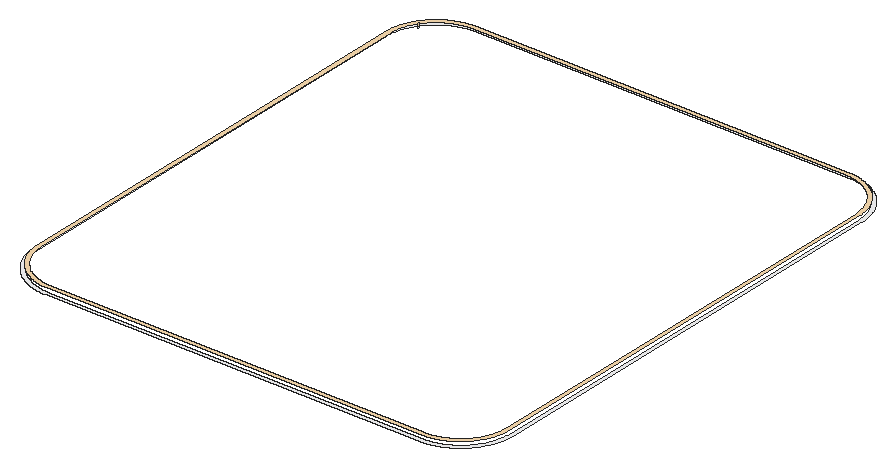
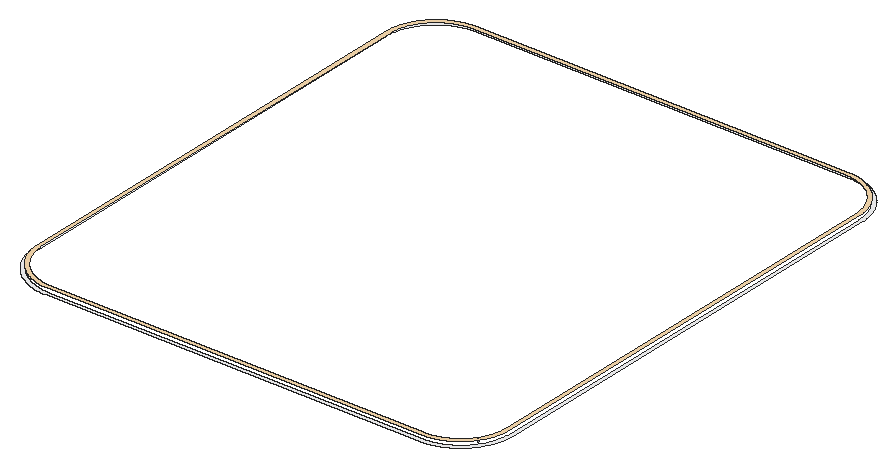
# SketchUp Ruby script. Lengths in inches.
U = 1.inch
M = Sketchup.active_model
def pt(a) = Geom::Point3d.new(a.map { |v| v * U })
def face(e, loops, mat)
  f = e.add_face(loops[0].map { |a| pt(a) })
  loops[1..].each { |l| e.add_face(l.map { |a| pt(a) }).erase! }
  f.material = f.back_material = mat if mat
  f
end
# faces: each face lists its corners as indices into pts; further lists are holes
def faces(e, pts, list, mat = nil) = list.each { |f| face(e, (f[0].is_a?(Array) ? f : [f]).map { |l| l.map { |i| pts[i] } }, mat) }
# xy, xz, yz: faces in a plane at the given z, y or x. An outline is a flat list of corners, or four numbers for a rectangle; further outlines are holes
def ring(l) = l.size == 4 ? [[l[0], l[1]], [l[2], l[1]], [l[2], l[3]], [l[0], l[3]]] : l.each_slice(2).to_a
def flat(e, list, mat, &to3) = list.each { |f| face(e, (f[0].is_a?(Array) ? f : [f]).map { |l| ring(l).map { |u, v| to3.(u, v) } }, mat) }
def xy(e, z, list, mat = nil) = flat(e, list, mat) { |x, y| [x, y, z] }
def xz(e, y, list, mat = nil) = flat(e, list, mat) { |x, z| [x, y, z] }
def yz(e, x, list, mat = nil) = flat(e, list, mat) { |y, z| [x, y, z] }
def lines(e, pts, list) = list.each { |a, b| e.add_line(pt(pts[a]), pt(pts[b])) }
# prism: a flat outline (further loops are holes) pulled along v
def prism(e, loops, v, mat = nil)
  f = face(e, loops, mat); d = Geom::Vector3d.new(v.map { |x| x * U })
  f.pushpull(f.normal.samedirection?(d) ? d.length : -d.length)
end
def box(e, o, s, mat = nil) = prism(e, [[o, [o[0] + s[0], o[1], o[2]], [o[0] + s[0], o[1] + s[1], o[2]], [o[0], o[1] + s[1], o[2]]]], [0, 0, s[2]], mat)
def at(x, y, z, deg = 0) = Geom::Transformation.translation(pt([x, y, z])) * Geom::Transformation.rotation(ORIGIN, Z_AXIS, deg.degrees)
def axes(o, x, y, z) = Geom::Transformation.new([*x, 0, *y, 0, *z, 0, *pt(o).to_a, 1])
def part(name) = M.definitions.add(name)
# library, detail: a bought-in or finely detailed component or shape, given as its bounding box
def library(name, o, s) = part(name).tap { |d| box(d.entities, o, s) }
def detail(e, o, s) = box(e.add_group.entities, o, s)
def put(e, d, t, mat = nil) = e.add_instance(d, t).tap { |i| i.material = mat if mat }
def group(e, t, mat = nil) = e.add_group.tap { |g| g.transformation = t; g.material = mat if mat }.entities
root = M.entities
M.materials.add("False Ceiling Light").color = [254, 223, 179]
M.materials.add("[Quartz Light Grey]").color = [251, 251, 252]
xy(root,115.32,[[[56.8,62.5,165.2,62.5,165.41,62.51,165.61,62.51,165.8125,62.52,166.01,62.53,166.22,62.55,166.42,62.56,166.62,62.58,166.82,62.61,167.02,62.63,167.42,62.69,167.625,62.72,167.82,62.76,168.42,62.88,168.82,62.98,169.01,63.03,169.21,63.08,169.4,63.14,169.6,63.2,169.98,63.32,170.74,63.6,171.12,63.76,171.3,63.84,171.49,63.92,171.67,64.01,171.86,64.1,172.04,64.1875,172.22,64.28,172.4,64.38,172.57,64.48,172.93,64.68,173.1,64.78,173.61,65.11,173.78,65.23,173.95,65.34,174.27,65.58,174.4375,65.7,174.75,65.95,175.07,66.21,175.22,66.35,175.37,66.48,175.82,66.9,176.1,67.18,176.52,67.63,176.65,67.78,176.79,67.93,177.05,68.25,177.3,68.5625,177.42,68.73,177.66,69.05,177.77,69.22,177.89,69.39,178.22,69.9,178.32,70.07,178.52,70.43,178.62,70.6,178.72,70.78,178.8125,70.96,178.9,71.14,178.99,71.33,179.08,71.51,179.16,71.7,179.24,71.88,179.4,72.26,179.68,73.02,179.8,73.4,179.86,73.6,179.92,73.79,179.97,73.99,180.02,74.18,180.12,74.58,180.24,75.18,180.28,75.375,180.31,75.58,180.37,75.98,180.39,76.18,180.42,76.38,180.44,76.58,180.45,76.78,180.47,76.99,180.48,77.1875,180.49,77.39,180.49,77.59,180.5,77.8,180.5,204.2,180.49,204.41,180.49,204.61,180.48,204.8125,180.47,205.01,180.45,205.22,180.44,205.42,180.42,205.62,180.39,205.82,180.37,206.02,180.31,206.42,180.28,206.625,180.24,206.82,180.12,207.42,180.02,207.82,179.97,208.01,179.92,208.21,179.86,208.4,179.8,208.6,179.68,208.98,179.4,209.74,179.24,210.12,179.16,210.3,179.08,210.49,178.99,210.67,178.9,210.86,178.8125,211.04,178.72,211.22,178.62,211.4,178.52,211.57,178.32,211.93,178.22,212.1,177.89,212.61,177.77,212.78,177.66,212.95,177.42,213.27,177.3,213.4375,177.05,213.75,176.79,214.07,176.65,214.22,176.52,214.37,176.1,214.82,175.82,215.1,175.37,215.52,175.22,215.65,175.07,215.79,174.75,216.05,174.4375,216.3,174.27,216.42,173.95,216.66,173.78,216.77,173.61,216.89,173.1,217.22,172.93,217.32,172.57,217.52,172.4,217.62,172.22,217.72,172.04,217.8125,171.86,217.9,171.67,217.99,171.49,218.08,171.3,218.16,171.12,218.24,170.74,218.4,169.98,218.68,169.6,218.8,169.4,218.86,169.21,218.92,169.01,218.97,168.82,219.02,168.42,219.12,167.82,219.24,167.625,219.28,167.42,219.31,167.02,219.37,166.82,219.39,166.62,219.42,166.42,219.44,166.22,219.45,166.01,219.47,165.8125,219.48,165.61,219.49,165.41,219.49,165.2,219.5,56.8,219.5,56.59,219.49,56.39,219.49,56.1875,219.48,55.99,219.47,55.78,219.45,55.58,219.44,55.38,219.42,55.18,219.39,54.98,219.37,54.58,219.31,54.375,219.28,54.18,219.24,53.58,219.12,53.18,219.02,52.99,218.97,52.79,218.92,52.6,218.86,52.4,218.8,52.02,218.68,51.26,218.4,50.88,218.24,50.7,218.16,50.51,218.08,50.33,217.99,50.14,217.9,49.96,217.8125,49.78,217.72,49.6,217.62,49.43,217.52,49.07,217.32,48.9,217.22,48.39,216.89,48.22,216.77,48.05,216.66,47.73,216.42,47.5625,216.3,47.25,216.05,46.93,215.79,46.78,215.65,46.63,215.52,46.18,215.1,45.9,214.82,45.48,214.37,45.35,214.22,45.21,214.07,44.95,213.75,44.7,213.4375,44.58,213.27,44.34,212.95,44.23,212.78,44.11,212.61,43.78,212.1,43.68,211.93,43.48,211.57,43.38,211.4,43.28,211.22,43.1875,211.04,43.1,210.86,43.01,210.67,42.92,210.49,42.84,210.3,42.76,210.12,42.6,209.74,42.32,208.98,42.2,208.6,42.14,208.4,42.08,208.21,42.03,208.01,41.98,207.82,41.88,207.42,41.76,206.82,41.72,206.625,41.69,206.42,41.63,206.02,41.61,205.82,41.58,205.62,41.56,205.42,41.55,205.22,41.53,205.01,41.52,204.8125,41.51,204.61,41.51,204.41,41.5,204.2,41.5,77.67,41.52,77.27,41.53,77.0625,41.54,76.86,41.58,76.46,41.6,76.25,41.62,76.05,41.71,75.45,41.75,75.25,41.78,75.05,41.82,74.85,41.87,74.65,41.91,74.45,42.01,74.05,42.0625,73.86,42.12,73.66,42.18,73.47,42.24,73.27,42.3,73.08,42.37,72.89,42.4375,72.69,42.51,72.5,42.58,72.3125,42.66,72.125,42.73,71.9375,42.82,71.75,42.9,71.5625,42.98,71.38,43.07,71.2,43.16,71.01,43.26,70.83,43.35,70.65,43.45,70.47,43.55,70.3,43.65,70.12,43.76,69.95,43.86,69.77,44.08,69.43,44.2,69.26,44.3125,69.09,44.43,68.93,44.55,68.76,44.67,68.6,44.93,68.28,45.05,68.125,45.18,67.97,45.32,67.8125,45.45,67.66,45.87,67.21,46.01,67.07,46.16,66.93,46.3,66.78,46.45,66.64,46.6,66.51,46.75,66.37,46.91,66.24,47.0625,66.11,47.22,65.98,47.375,65.85,47.54,65.72,47.86,65.48,48.2,65.24,48.36,65.13,48.7,64.91,48.88,64.8,49.05,64.69,49.23,64.59,49.4,64.49,49.76,64.29,49.94,64.2,50.31,64.02,50.49,63.93,50.68,63.85,50.86,63.77,51.05,63.6875,51.24,63.61,51.43,63.54,51.62,63.46,51.81,63.39,52,63.33,52.19,63.26,52.39,63.2,52.58,63.14,52.78,63.09,52.98,63.03,53.17,62.98,53.57,62.88,54.17,62.76,54.37,62.73,54.57,62.69,54.97,62.63,55.17,62.61,55.58,62.57,55.98,62.53,56.1875,62.52,56.39,62.51,56.59,62.51],[56.62,63.5,55.86,63.54,55.67,63.5625,55.48,63.58,55.29,63.6,54.91,63.65,54.72,63.68,54.54,63.71,54.35,63.74,54.16,63.78,53.98,63.82,53.6,63.9,53.42,63.95,53.23,64,52.87,64.1,52.6875,64.16,52.5,64.21,52.32,64.27,52.14,64.34,51.97,64.4,51.43,64.61,51.26,64.69,51.08,64.76,50.74,64.92,50.57,65.01,50.4,65.09,49.89,65.36,49.73,65.46,49.5625,65.55,49.4,65.65,49.08,65.85,48.76,66.07,48.61,66.18,48.45,66.29,48.3,66.4,48.15,66.52,48,66.63,47.85,66.75,47.7,66.875,47.56,67,47.41,67.12,47.27,67.25,47.13,67.375,46.99,67.51,46.86,67.64,46.72,67.77,46.46,68.05,46.33,68.1875,46.2,68.33,46.07,68.47,45.95,68.61,45.82,68.76,45.7,68.91,45.59,69.06,45.35,69.36,45.24,69.51,45.02,69.83,44.92,69.98,44.8125,70.14,44.71,70.3,44.61,70.47,44.51,70.63,44.42,70.79,44.32,70.96,44.23,71.125,44.14,71.3,43.97,71.64,43.73,72.15,43.66,72.33,43.58,72.5,43.44,72.86,43.375,73.04,43.25,73.4,43.13,73.76,43.08,73.94,42.98,74.31,42.93,74.49,42.89,74.68,42.84,74.86,42.8,75.05,42.77,75.24,42.73,75.42,42.61,76.18,42.59,76.37,42.57,76.55,42.55,76.74,42.54,76.93,42.53,77.125,42.51,77.5,42.5,77.7,42.5,204.38,42.54,205.14,42.5625,205.33,42.58,205.52,42.6,205.7,42.65,206.08,42.71,206.46,42.74,206.64,42.78,206.83,42.82,207.01,42.86,207.2,42.9,207.38,42.95,207.57,42.99,207.75,43.04,207.9375,43.1,208.12,43.15,208.3,43.33,208.84,43.4,209.02,43.46,209.2,43.6,209.55,43.68,209.72,43.75,209.9,43.91,210.24,44,210.41,44.08,210.58,44.35,211.09,44.44,211.25,44.54,211.41,44.64,211.58,44.94,212.06,45.05,212.21,45.16,212.37,45.27,212.52,45.38,212.68,45.5,212.83,45.61,212.98,45.85,213.27,45.97,213.42,46.1,213.5625,46.22,213.7,46.61,214.12,46.75,214.25,46.88,214.39,47.3,214.78,47.4375,214.9,47.58,215.03,47.73,215.15,48.02,215.39,48.17,215.5,48.32,215.62,48.48,215.73,48.63,215.84,48.79,215.95,48.94,216.06,49.42,216.36,49.59,216.46,49.75,216.56,49.91,216.65,50.42,216.92,50.59,217,50.76,217.09,51.1,217.25,51.28,217.32,51.45,217.4,51.8,217.54,51.98,217.6,52.16,217.67,52.7,217.85,52.88,217.9,53.0625,217.96,53.25,218.01,53.43,218.05,53.62,218.1,53.8,218.14,53.99,218.18,54.17,218.22,54.36,218.26,54.54,218.29,54.92,218.35,55.3,218.4,55.48,218.42,55.67,218.4375,55.86,218.46,56.62,218.5,165.38,218.5,166.14,218.46,166.33,218.4375,166.52,218.42,166.7,218.4,167.08,218.35,167.46,218.29,167.64,218.26,167.83,218.22,168.01,218.18,168.2,218.14,168.38,218.1,168.57,218.05,168.75,218.01,168.9375,217.96,169.12,217.9,169.3,217.85,169.84,217.67,170.02,217.6,170.2,217.54,170.55,217.4,170.72,217.32,170.9,217.25,171.24,217.09,171.41,217,171.58,216.92,172.09,216.65,172.25,216.56,172.41,216.46,172.58,216.36,173.06,216.06,173.21,215.95,173.37,215.84,173.52,215.73,173.68,215.62,173.83,215.5,173.98,215.39,174.27,215.15,174.42,215.03,174.5625,214.9,174.7,214.78,175.12,214.39,175.25,214.25,175.39,214.12,175.78,213.7,175.9,213.5625,176.03,213.42,176.15,213.27,176.39,212.98,176.5,212.83,176.62,212.68,176.73,212.52,176.84,212.37,176.95,212.21,177.06,212.06,177.36,211.58,177.46,211.41,177.56,211.25,177.65,211.09,177.92,210.58,178,210.41,178.09,210.24,178.25,209.9,178.32,209.72,178.4,209.55,178.54,209.2,178.6,209.02,178.67,208.84,178.85,208.3,178.9,208.12,178.96,207.9375,179.01,207.75,179.05,207.57,179.1,207.38,179.14,207.2,179.18,207.01,179.22,206.83,179.26,206.64,179.29,206.46,179.35,206.08,179.4,205.7,179.42,205.52,179.4375,205.33,179.46,205.14,179.5,204.38,179.5,77.62,179.46,76.86,179.4375,76.67,179.42,76.48,179.4,76.3,179.35,75.92,179.29,75.54,179.26,75.36,179.22,75.17,179.18,74.99,179.14,74.8,179.1,74.62,179.05,74.43,179.01,74.25,178.96,74.0625,178.9,73.88,178.85,73.7,178.67,73.16,178.6,72.98,178.54,72.8,178.4,72.45,178.32,72.28,178.25,72.1,178.09,71.76,178,71.59,177.92,71.42,177.65,70.91,177.56,70.75,177.46,70.59,177.36,70.42,177.06,69.94,176.95,69.79,176.84,69.63,176.73,69.48,176.62,69.32,176.5,69.17,176.39,69.02,176.15,68.73,176.03,68.58,175.9,68.4375,175.78,68.3,175.39,67.88,175.25,67.75,175.12,67.61,174.7,67.22,174.5625,67.1,174.42,66.97,174.27,66.85,173.98,66.61,173.83,66.5,173.68,66.38,173.52,66.27,173.37,66.16,173.21,66.05,173.06,65.94,172.58,65.64,172.41,65.54,172.25,65.44,172.09,65.35,171.58,65.08,171.41,65,171.24,64.91,170.9,64.75,170.72,64.68,170.55,64.6,170.2,64.46,170.02,64.4,169.84,64.33,169.3,64.15,169.12,64.1,168.9375,64.04,168.75,63.99,168.57,63.95,168.38,63.9,168.2,63.86,168.01,63.82,167.83,63.78,167.64,63.74,167.46,63.71,167.08,63.65,166.7,63.6,166.52,63.58,166.33,63.5625,166.14,63.54,165.38,63.5]]],"[Quartz Light Grey]")
xy(root,116.49,[[[56.62,63.5,165.38,63.5,166.14,63.54,166.33,63.5625,166.52,63.58,166.7,63.6,167.08,63.65,167.46,63.71,167.64,63.74,167.83,63.78,168.01,63.82,168.2,63.86,168.38,63.9,168.57,63.95,168.75,63.99,168.9375,64.04,169.12,64.1,169.3,64.15,169.84,64.33,170.02,64.4,170.2,64.46,170.55,64.6,170.72,64.68,170.9,64.75,171.24,64.91,171.41,65,171.58,65.08,172.09,65.35,172.25,65.44,172.41,65.54,172.58,65.64,173.06,65.94,173.21,66.05,173.37,66.16,173.52,66.27,173.68,66.38,173.83,66.5,173.98,66.61,174.27,66.85,174.42,66.97,174.5625,67.1,174.7,67.22,175.12,67.61,175.25,67.75,175.39,67.88,175.78,68.3,175.9,68.4375,176.03,68.58,176.15,68.73,176.39,69.02,176.5,69.17,176.62,69.32,176.73,69.48,176.84,69.63,176.95,69.79,177.06,69.94,177.36,70.42,177.46,70.59,177.56,70.75,177.65,70.91,177.92,71.42,178,71.59,178.09,71.76,178.25,72.1,178.32,72.28,178.4,72.45,178.54,72.8,178.6,72.98,178.67,73.16,178.85,73.7,178.9,73.88,178.96,74.0625,179.01,74.25,179.05,74.43,179.1,74.62,179.14,74.8,179.18,74.99,179.22,75.17,179.26,75.36,179.29,75.54,179.35,75.92,179.4,76.3,179.42,76.48,179.4375,76.67,179.46,76.86,179.5,77.62,179.5,204.38,179.46,205.14,179.4375,205.33,179.42,205.52,179.4,205.7,179.35,206.08,179.29,206.46,179.26,206.64,179.22,206.83,179.18,207.01,179.14,207.2,179.1,207.38,179.05,207.57,179.01,207.75,178.96,207.9375,178.9,208.12,178.85,208.3,178.67,208.84,178.6,209.02,178.54,209.2,178.4,209.55,178.32,209.72,178.25,209.9,178.09,210.24,178,210.41,177.92,210.58,177.65,211.09,177.56,211.25,177.46,211.41,177.36,211.58,177.06,212.06,176.95,212.21,176.84,212.37,176.73,212.52,176.62,212.68,176.5,212.83,176.39,212.98,176.15,213.27,176.03,213.42,175.9,213.5625,175.78,213.7,175.39,214.12,175.25,214.25,175.12,214.39,174.7,214.78,174.5625,214.9,174.42,215.03,174.27,215.15,173.98,215.39,173.83,215.5,173.68,215.62,173.52,215.73,173.37,215.84,173.21,215.95,173.06,216.06,172.58,216.36,172.41,216.46,172.25,216.56,172.09,216.65,171.58,216.92,171.41,217,171.24,217.09,170.9,217.25,170.72,217.32,170.55,217.4,170.2,217.54,170.02,217.6,169.84,217.67,169.3,217.85,169.12,217.9,168.9375,217.96,168.75,218.01,168.57,218.05,168.38,218.1,168.2,218.14,168.01,218.18,167.83,218.22,167.64,218.26,167.46,218.29,167.08,218.35,166.7,218.4,166.52,218.42,166.33,218.4375,166.14,218.46,165.38,218.5,56.62,218.5,55.86,218.46,55.67,218.4375,55.48,218.42,55.3,218.4,54.92,218.35,54.54,218.29,54.36,218.26,54.17,218.22,53.99,218.18,53.8,218.14,53.62,218.1,53.43,218.05,53.25,218.01,53.0625,217.96,52.88,217.9,52.7,217.85,52.16,217.67,51.98,217.6,51.8,217.54,51.45,217.4,51.28,217.32,51.1,217.25,50.76,217.09,50.59,217,50.42,216.92,49.91,216.65,49.75,216.56,49.59,216.46,49.42,216.36,48.94,216.06,48.79,215.95,48.63,215.84,48.48,215.73,48.32,215.62,48.17,215.5,48.02,215.39,47.73,215.15,47.58,215.03,47.4375,214.9,47.3,214.78,46.88,214.39,46.75,214.25,46.61,214.12,46.22,213.7,46.1,213.5625,45.97,213.42,45.85,213.27,45.61,212.98,45.5,212.83,45.38,212.68,45.27,212.52,45.16,212.37,45.05,212.21,44.94,212.06,44.64,211.58,44.54,211.41,44.44,211.25,44.35,211.09,44.08,210.58,44,210.41,43.91,210.24,43.75,209.9,43.68,209.72,43.6,209.55,43.46,209.2,43.4,209.02,43.33,208.84,43.15,208.3,43.1,208.12,43.04,207.9375,42.99,207.75,42.95,207.57,42.9,207.38,42.86,207.2,42.82,207.01,42.78,206.83,42.74,206.64,42.71,206.46,42.65,206.08,42.6,205.7,42.58,205.52,42.5625,205.33,42.54,205.14,42.5,204.38,42.5,77.7,42.51,77.5,42.53,77.125,42.54,76.93,42.55,76.74,42.57,76.55,42.59,76.37,42.61,76.18,42.73,75.42,42.77,75.24,42.8,75.05,42.84,74.86,42.89,74.68,42.93,74.49,42.98,74.31,43.08,73.94,43.13,73.76,43.25,73.4,43.375,73.04,43.44,72.86,43.58,72.5,43.66,72.33,43.73,72.15,43.97,71.64,44.14,71.3,44.23,71.125,44.32,70.96,44.42,70.79,44.51,70.63,44.61,70.47,44.71,70.3,44.8125,70.14,44.92,69.98,45.02,69.83,45.24,69.51,45.35,69.36,45.59,69.06,45.7,68.91,45.82,68.76,45.95,68.61,46.07,68.47,46.2,68.33,46.33,68.1875,46.46,68.05,46.72,67.77,46.86,67.64,46.99,67.51,47.13,67.375,47.27,67.25,47.41,67.12,47.56,67,47.7,66.875,47.85,66.75,48,66.63,48.15,66.52,48.3,66.4,48.45,66.29,48.61,66.18,48.76,66.07,49.08,65.85,49.4,65.65,49.5625,65.55,49.73,65.46,49.89,65.36,50.4,65.09,50.57,65.01,50.74,64.92,51.08,64.76,51.26,64.69,51.43,64.61,51.97,64.4,52.14,64.34,52.32,64.27,52.5,64.21,52.6875,64.16,52.87,64.1,53.23,64,53.42,63.95,53.6,63.9,53.98,63.82,54.16,63.78,54.35,63.74,54.54,63.71,54.72,63.68,54.91,63.65,55.29,63.6,55.48,63.58,55.67,63.5625,55.86,63.54],[56.65,64.5,56.11,64.53,55.9375,64.54,55.76,64.56,55.58,64.57,55.41,64.59,55.23,64.62,55.06,64.64,54.88,64.67,54.71,64.7,54.53,64.73,54.36,64.76,54.18,64.8,54.01,64.84,53.84,64.875,53.67,64.92,53.49,64.96,52.98,65.11,52.81,65.17,52.65,65.22,52.48,65.28,52.3125,65.34,52.15,65.4,51.98,65.47,51.82,65.53,51.65,65.6,51.49,65.67,51.33,65.75,51.17,65.82,50.85,65.98,50.69,66.0625,50.54,66.15,50.38,66.23,49.93,66.5,49.77,66.6,49.625,66.69,49.48,66.79,49.33,66.89,49.1875,66.99,49.04,67.09,48.34,67.64,48.21,67.76,48.07,67.87,47.94,67.99,47.8125,68.11,47.68,68.23,47.55,68.35,47.43,68.48,47.18,68.73,47.0625,68.86,46.94,68.99,46.82,69.13,46.71,69.26,46.6,69.4,46.48,69.54,46.375,69.67,46.26,69.8125,46.16,69.96,46.05,70.1,45.95,70.24,45.75,70.54,45.65,70.68,45.56,70.83,45.47,70.99,45.375,71.14,45.29,71.29,45.2,71.45,45.11,71.6,44.95,71.92,44.87,72.07,44.79,72.23,44.72,72.39,44.65,72.56,44.51,72.88,44.44,73.05,44.38,73.21,44.26,73.55,44.2,73.71,44.14,73.88,43.99,74.39,43.94,74.5625,43.9,74.73,43.86,74.91,43.78,75.25,43.75,75.43,43.71,75.6,43.68,75.78,43.66,75.95,43.63,76.125,43.61,76.3,43.59,76.48,43.57,76.65,43.55,76.83,43.54,77.01,43.52,77.18,43.51,77.36,43.51,77.54,43.5,77.72,43.5,204.35,43.52,204.71,43.53,204.88,43.54,205.06,43.56,205.24,43.57,205.41,43.59,205.59,43.62,205.76,43.64,205.9375,43.67,206.11,43.69,206.29,43.73,206.46,43.76,206.63,43.79,206.81,43.87,207.15,43.92,207.32,43.96,207.49,44.16,208.17,44.22,208.34,44.27,208.51,44.33,208.67,44.4,208.84,44.46,209,44.53,209.17,44.74,209.65,44.82,209.8125,44.89,209.97,45.05,210.29,45.14,210.44,45.22,210.6,45.58,211.2,45.78,211.5,45.875,211.65,45.98,211.79,46.08,211.94,46.18,212.08,46.51,212.5,46.62,212.63,46.73,212.77,47.45,213.55,48.23,214.27,48.37,214.38,48.5,214.49,48.92,214.82,49.06,214.92,49.21,215.02,49.35,215.125,49.5,215.22,49.8,215.42,50.4,215.78,50.56,215.86,50.71,215.95,51.03,216.11,51.1875,216.18,51.35,216.26,51.83,216.47,52,216.54,52.16,216.6,52.33,216.67,52.49,216.73,52.66,216.78,52.83,216.84,53.51,217.04,53.68,217.08,53.85,217.13,54.19,217.21,54.37,217.24,54.54,217.27,54.71,217.31,54.89,217.33,55.0625,217.36,55.24,217.38,55.41,217.41,55.59,217.43,55.76,217.44,55.94,217.46,56.12,217.47,56.29,217.48,56.65,217.5,165.35,217.5,165.71,217.48,165.88,217.47,166.06,217.46,166.24,217.44,166.41,217.43,166.59,217.41,166.76,217.38,166.9375,217.36,167.11,217.33,167.29,217.31,167.46,217.27,167.63,217.24,167.81,217.21,168.15,217.13,168.32,217.08,168.49,217.04,169.17,216.84,169.34,216.78,169.51,216.73,169.67,216.67,169.84,216.6,170,216.54,170.17,216.47,170.65,216.26,170.8125,216.18,170.97,216.11,171.29,215.95,171.44,215.86,171.6,215.78,172.2,215.42,172.5,215.22,172.65,215.125,172.79,215.02,172.94,214.92,173.08,214.82,173.5,214.49,173.63,214.38,173.77,214.27,174.55,213.55,175.27,212.77,175.38,212.63,175.49,212.5,175.82,212.08,175.92,211.94,176.02,211.79,176.125,211.65,176.22,211.5,176.42,211.2,176.78,210.6,176.86,210.44,176.95,210.29,177.11,209.97,177.18,209.8125,177.26,209.65,177.47,209.17,177.54,209,177.6,208.84,177.67,208.67,177.73,208.51,177.78,208.34,177.84,208.17,178.04,207.49,178.08,207.32,178.13,207.15,178.21,206.81,178.24,206.63,178.27,206.46,178.31,206.29,178.33,206.11,178.36,205.9375,178.38,205.76,178.41,205.59,178.43,205.41,178.44,205.24,178.46,205.06,178.47,204.88,178.48,204.71,178.5,204.35,178.5,77.65,178.48,77.29,178.47,77.12,178.46,76.94,178.44,76.76,178.43,76.59,178.41,76.41,178.38,76.24,178.36,76.0625,178.33,75.89,178.31,75.71,178.27,75.54,178.24,75.37,178.21,75.19,178.13,74.85,178.08,74.68,178.04,74.51,177.84,73.83,177.78,73.66,177.73,73.49,177.67,73.33,177.6,73.16,177.54,73,177.47,72.83,177.26,72.35,177.18,72.1875,177.11,72.03,176.95,71.71,176.86,71.56,176.78,71.4,176.42,70.8,176.22,70.5,176.125,70.35,176.02,70.21,175.92,70.06,175.82,69.92,175.49,69.5,175.38,69.37,175.27,69.23,174.55,68.45,173.77,67.73,173.63,67.62,173.5,67.51,173.08,67.18,172.94,67.08,172.79,66.98,172.65,66.875,172.5,66.78,172.2,66.58,171.6,66.22,171.44,66.14,171.29,66.05,170.97,65.89,170.8125,65.82,170.65,65.74,170.17,65.53,170,65.46,169.84,65.4,169.67,65.33,169.51,65.27,169.34,65.22,169.17,65.16,168.49,64.96,168.32,64.92,168.15,64.87,167.81,64.79,167.63,64.76,167.46,64.73,167.29,64.69,167.11,64.67,166.9375,64.64,166.76,64.62,166.59,64.59,166.41,64.57,166.24,64.56,166.06,64.54,165.88,64.53,165.71,64.52,165.35,64.5]]],"False Ceiling Light")
p = [[45.78,211.5,115.32],[45.875,211.65,115.32],[45.875,211.65,116.49],[45.78,211.5,116.49],[45.875,211.65,115.32],[45.78,211.5,115.32],
  [45.78,211.5,115.91],[45.875,211.65,115.91]]
faces(root,p,[[0,1,2,3]],"False Ceiling Light")
faces(root,p,[[4,5,6,7]],"[Quartz Light Grey]")
